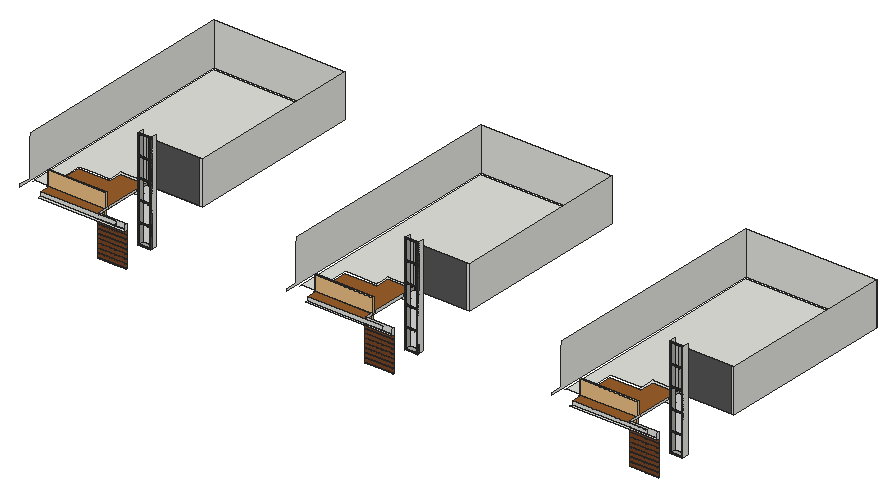
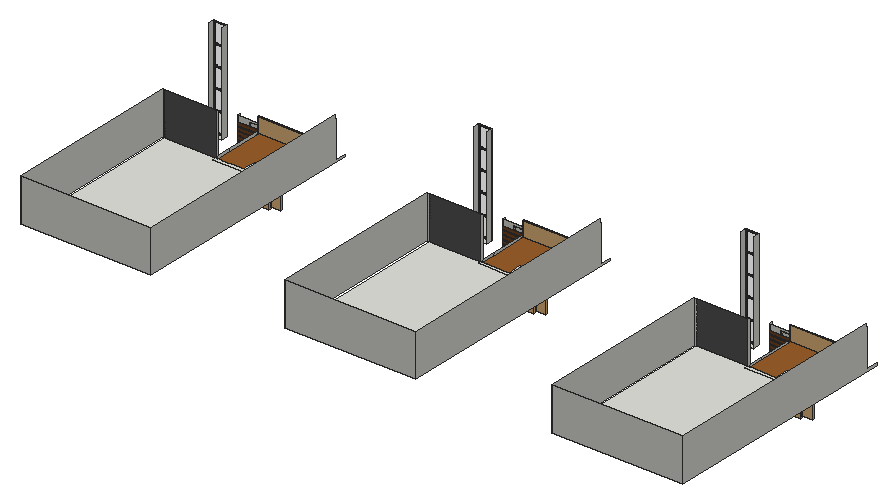
# SketchUp Ruby script. Lengths in inches.
U = 1.inch
M = Sketchup.active_model
def pt(a) = Geom::Point3d.new(a.map { |v| v * U })
def face(e, loops, mat)
  f = e.add_face(loops[0].map { |a| pt(a) })
  loops[1..].each { |l| e.add_face(l.map { |a| pt(a) }).erase! }
  f.material = f.back_material = mat if mat
  f
end
# faces: each face lists its corners as indices into pts; further lists are holes
def faces(e, pts, list, mat = nil) = list.each { |f| face(e, (f[0].is_a?(Array) ? f : [f]).map { |l| l.map { |i| pts[i] } }, mat) }
# xy, xz, yz: faces in a plane at the given z, y or x. An outline is a flat list of corners, or four numbers for a rectangle; further outlines are holes
def ring(l) = l.size == 4 ? [[l[0], l[1]], [l[2], l[1]], [l[2], l[3]], [l[0], l[3]]] : l.each_slice(2).to_a
def flat(e, list, mat, &to3) = list.each { |f| face(e, (f[0].is_a?(Array) ? f : [f]).map { |l| ring(l).map { |u, v| to3.(u, v) } }, mat) }
def xy(e, z, list, mat = nil) = flat(e, list, mat) { |x, y| [x, y, z] }
def xz(e, y, list, mat = nil) = flat(e, list, mat) { |x, z| [x, y, z] }
def yz(e, x, list, mat = nil) = flat(e, list, mat) { |y, z| [x, y, z] }
def lines(e, pts, list) = list.each { |a, b| e.add_line(pt(pts[a]), pt(pts[b])) }
# prism: a flat outline (further loops are holes) pulled along v
def prism(e, loops, v, mat = nil)
  f = face(e, loops, mat); d = Geom::Vector3d.new(v.map { |x| x * U })
  f.pushpull(f.normal.samedirection?(d) ? d.length : -d.length)
end
def box(e, o, s, mat = nil) = prism(e, [[o, [o[0] + s[0], o[1], o[2]], [o[0] + s[0], o[1] + s[1], o[2]], [o[0], o[1] + s[1], o[2]]]], [0, 0, s[2]], mat)
def at(x, y, z, deg = 0) = Geom::Transformation.translation(pt([x, y, z])) * Geom::Transformation.rotation(ORIGIN, Z_AXIS, deg.degrees)
def axes(o, x, y, z) = Geom::Transformation.new([*x, 0, *y, 0, *z, 0, *pt(o).to_a, 1])
def part(name) = M.definitions.add(name)
# library, detail: a bought-in or finely detailed component or shape, given as its bounding box
def library(name, o, s) = part(name).tap { |d| box(d.entities, o, s) }
def detail(e, o, s) = box(e.add_group.entities, o, s)
def put(e, d, t, mat = nil) = e.add_instance(d, t).tap { |i| i.material = mat if mat }
def group(e, t, mat = nil) = e.add_group.tap { |g| g.transformation = t; g.material = mat if mat }.entities
root = M.entities
M.materials.add("Aluminum_Polished").color = [83, 85, 85]
M.materials.add("Glass_Window_Neutral").color = [0, 0, 0]
M.materials["Glass_Window_Neutral"].alpha = 0.125
M.materials.add("[Color M04]").color = [142, 142, 142]
M.materials.add("[Color M06]").color = [86, 86, 86]
M.materials.add("[Wood Floor Dark]").color = [153, 94, 42]
M.materials.add("[Wood Veneer 01]").color = [120, 70, 37]
c1 = library("Group\#1",[0,0,0],[29.75,5.78,110.95])
c2 = part("Group\#54")
box(c2.entities,[0,0,0],[2,1,28])
c3 = part("Group\#56")
p = [[0.11,0.32,0.14],[0.11,0.69,0.14]]
lines(c3.entities,p,[[0,1]])
g1 = group(c3.entities,at(0.11,0,0))
prism(g1,[[[0,0.24,0],[0,0.32,0.14],[0,0.24,0.27],[0,0.08,0.27],[0,0,0.14],[0,0.08,0]]],[-0.11,0,0])
c4 = part("Ver Glass Railing")
g2 = group(c4.entities,at(0,0,0),"Aluminum_Polished")
box(g2,[0,0,0],[2,185,2])
g3 = group(c4.entities,at(0,0,2),"Aluminum_Polished")
p = [[1.41,1,0],[1.41,36.8,0],[1.41,184,0],[1.29,184,0],[1.29,1,0],[1.29,36.8,0],
  [1.41,184,28],[1.29,184,28],[1.41,148.2,28],[1.29,148.2,28],[1.41,1,28],[1.29,1,28],
  [1.29,111.4,28],[1.29,111.4,0],[1.41,111.4,0],[1.41,111.4,28],[1.29,110.4,0],[1.29,110.4,28],
  [1.41,110.4,28],[1.41,110.4,0],[1.29,74.6,28],[1.29,74.6,0],[1.41,74.6,0],[1.41,74.6,28],
  [1.29,73.6,0],[1.29,73.6,28],[1.41,73.6,28],[1.41,73.6,0],[1.29,148.2,0],[1.41,148.2,0],
  [1.29,147.2,0],[1.29,147.2,28],[1.41,147.2,28],[1.41,147.2,0],[1.29,37.8,28],[1.29,37.8,0],
  [1.41,37.8,0],[1.41,37.8,28],[1.29,36.8,28],[1.41,36.8,28]]
lines(g3,p,[[0,1],[2,3],[4,5],[6,7],[6,8],[7,9],[10,11],[2,6],[3,7],[0,4],[11,4],[10,0],
  [12,13],[14,15],[16,17],[18,19],[20,21],[22,23],[24,25],[26,27],[27,22],[24,21],[23,26],[20,25],
  [9,28],[29,8],[30,31],[32,33],[33,29],[30,28],[8,32],[9,31],[34,35],[36,37],[5,38],[39,1],
  [1,36],[5,35],[37,39],[14,33],[19,14],[22,19],[36,27],[13,30],[16,13],[21,16],[35,24],[15,18],
  [12,17],[29,2],[28,3],[18,23],[32,15],[17,20],[31,12],[26,37],[25,34],[34,38],[39,10],[38,11]])
g4 = group(g3,at(1.79,1,0))
box(g4,[-0.5,0,0],[0.125,183,28],"Glass_Window_Neutral")
g5 = group(g3,at(0,184,28))
box(g5,[0,-184,0],[2.5,185,1])
put(g3,c2,axes([2,185,28],[-1,0,0],[0,-1,0],[0,0,-1]))
put(g3,c2,axes([2,1,28],[-1,0,0],[0,-1,0],[0,0,-1]))
put(g3,c2,axes([2,111.4,28],[-1,0,0],[0,-1,0],[0,0,-1]))
put(g3,c2,axes([2,74.6,28],[-1,0,0],[0,-1,0],[0,0,-1]))
g6 = group(g3,at(2,148.2,28))
box(g6,[-2,-1,-28],[2,1,28])
put(g3,c2,axes([2,37.8,28],[-1,0,0],[0,-1,0],[0,0,-1]))
put(g3,c3,at(1.17,146.31,24.26))
put(g3,c3,axes([1.17,148.89,24.54],[1,0,0],[0,-1,0],[0,0,-1]))
put(g3,c3,axes([1.17,148.89,4.79],[1,0,0],[0,-1,0],[0,0,-1]))
put(g3,c3,at(1.17,146.31,4.51))
put(g3,c3,at(1.17,109.51,4.51))
put(g3,c3,axes([1.17,112.09,4.79],[1,0,0],[0,-1,0],[0,0,-1]))
put(g3,c3,axes([1.17,112.09,24.54],[1,0,0],[0,-1,0],[0,0,-1]))
put(g3,c3,at(1.17,109.51,24.26))
put(g3,c3,axes([1.17,75.29,24.54],[1,0,0],[0,-1,0],[0,0,-1]))
put(g3,c3,at(1.17,72.71,4.51))
put(g3,c3,axes([1.17,75.29,4.79],[1,0,0],[0,-1,0],[0,0,-1]))
put(g3,c3,at(1.17,72.71,24.26))
put(g3,c3,axes([1.17,38.49,24.54],[1,0,0],[0,-1,0],[0,0,-1]))
put(g3,c3,at(1.17,35.91,4.51))
put(g3,c3,axes([1.17,38.49,4.79],[1,0,0],[0,-1,0],[0,0,-1]))
put(g3,c3,at(1.17,35.91,24.26))
c5 = library("Glass Railing",[0,0,0],[139.5,4.76,42])
xy(root,154.375,[[1098.03,272.125,1148.06,273.0625],[1148.06,272.125,1181.97,273.0625],[1884.4,272.125,1934.43,273.0625],[1934.43,272.125,1968.34,273.0625],[2664.78,272.125,2714.81,273.0625],
  [2714.81,272.125,2748.72,273.0625]])
xy(root,155.86,[[1098.03,272.125,1181.97,273.0625],[1884.4,272.125,1968.34,273.0625],[2664.78,272.125,2748.72,273.0625]])
xy(root,167.1875,[[1098.03,272.125,1148.06,273.0625],[1148.06,272.125,1181.97,273.0625],[1884.4,272.125,1934.43,273.0625],[1934.43,272.125,1968.34,273.0625],[2664.78,272.125,2714.81,273.0625],
  [2714.81,272.125,2748.72,273.0625]])
xy(root,168.67,[[1098.03,272.125,1181.97,273.0625],[1884.4,272.125,1968.34,273.0625],[2664.78,272.125,2748.72,273.0625]])
xy(root,180,[[1098.03,272.125,1148.06,273.0625],[1148.06,272.125,1181.97,273.0625],[1884.4,272.125,1934.43,273.0625],[1934.43,272.125,1968.34,273.0625],[2664.78,272.125,2714.81,273.0625],
  [2714.81,272.125,2748.72,273.0625]])
xy(root,181.48,[[1098.03,272.125,1181.97,273.0625],[1884.4,272.125,1968.34,273.0625],[2664.78,272.125,2748.72,273.0625]])
xy(root,192.8125,[[1098.03,272.125,1148.06,273.0625],[1148.06,272.125,1181.97,273.0625],[1884.4,272.125,1934.43,273.0625],[1934.43,272.125,1968.34,273.0625],[2664.78,272.125,2714.81,273.0625],
  [2714.81,272.125,2748.72,273.0625]])
xy(root,194.3,[[1098.03,272.125,1181.97,273.0625],[1884.4,272.125,1968.34,273.0625],[2664.78,272.125,2748.72,273.0625]])
xy(root,205.625,[[1098.03,272.125,1148.06,273.0625],[1148.06,272.125,1181.97,273.0625],[1884.4,272.125,1934.43,273.0625],[1934.43,272.125,1968.34,273.0625],[2664.78,272.125,2714.81,273.0625],
  [2714.81,272.125,2748.72,273.0625]])
xy(root,207.11,[[1098.03,272.125,1181.97,273.0625],[1884.4,272.125,1968.34,273.0625],[2664.78,272.125,2748.72,273.0625]])
xy(root,217.36,[[1200.15,289.5,1239.03,308.24],[1986.53,289.5,2025.4,308.24],[2766.9,289.5,2805.78,308.24]])
xy(root,218.4375,[[1098.03,272.125,1148.06,273.0625],[1148.06,272.125,1181.97,273.0625],[1884.4,272.125,1934.43,273.0625],[1934.43,272.125,1968.34,273.0625],[2664.78,272.125,2714.81,273.0625],
  [2714.81,272.125,2748.72,273.0625]])
xy(root,219.92,[[1098.03,272.125,1181.97,273.0625],[1884.4,272.125,1968.34,273.0625],[2664.78,272.125,2748.72,273.0625]])
xy(root,231.25,[[1098.03,272.125,1148.06,273.0625],[1148.06,272.125,1181.97,273.0625],[1884.4,272.125,1934.43,273.0625],[1934.43,272.125,1968.34,273.0625],[2664.78,272.125,2714.81,273.0625],
  [2714.81,272.125,2748.72,273.0625]])
xy(root,231.75,[[1037.97,452.5625,1079.72,462.67],[1824.35,452.5625,1866.1,462.67],[2604.72,452.5625,2646.47,462.67]])
xy(root,232.73,[[1098.03,272.125,1181.97,273.0625],[1884.4,272.125,1968.34,273.0625],[2664.78,272.125,2748.72,273.0625]])
xy(root,244.0625,[[1098.03,272.125,1148.06,273.0625],[1148.06,272.125,1181.97,273.0625],[1884.4,272.125,1934.43,273.0625],[1934.43,272.125,1968.34,273.0625],[2664.78,272.125,2714.81,273.0625],
  [2714.81,272.125,2748.72,273.0625]])
xy(root,245.55,[[1098.03,272.125,1181.97,273.0625],[1884.4,272.125,1968.34,273.0625],[2664.78,272.125,2748.72,273.0625]])
xy(root,256.875,[[928.09,264.125,928.09,272.68,1098.03,272.98,1098.03,272.125,1181.97,272.125,1181.97,264.125],[1714.47,264.125,1714.47,272.68,1884.4,272.98,1884.4,272.125,1968.34,272.125,1968.34,264.125],[2494.84,264.125,2494.84,272.68,2664.78,272.98,2664.78,272.125,2748.72,272.125,2748.72,264.125],[1098.03,272.125,1098.03,272.98,1148.06,273.0625,1148.06,272.125],[1148.06,272.125,1181.97,273.0625],
  [1884.4,272.125,1884.4,272.98,1934.43,273.0625,1934.43,272.125],[1934.43,272.125,1968.34,273.0625],[2664.78,272.125,2664.78,272.98,2714.81,273.0625,2714.81,272.125],[2714.81,272.125,2748.72,273.0625],[1098.03,272.98,1148.06,273.0625,1098.03,273.0625],
  [1884.4,272.98,1934.43,273.0625,1884.4,273.0625],[2664.78,272.98,2714.81,273.0625,2664.78,273.0625]])
xy(root,267.625,[[881.96,308.24,922.07,308.24,922.07,421.04,971.61,421.04,1012.79,420.39,1012.79,462.67,1103.7,462.67,1103.7,452.5625,1253.34,452.5625,1253.34,968.69,881.96,968.69],[1668.33,308.24,1708.45,308.24,1708.45,421.04,1757.99,421.04,1799.16,420.39,1799.16,462.67,1890.08,462.67,1890.08,452.5625,2039.72,452.5625,2039.72,968.69,1668.33,968.69],[2448.71,308.24,2488.82,308.24,2488.82,421.04,2538.36,421.04,2579.54,420.39,2579.54,462.67,2670.45,462.67,2670.45,452.5625,2820.09,452.5625,2820.09,968.69,2448.71,968.69],[1012.79,411.0625,1019.84,411.0625,1019.84,452.5625,1103.7,452.5625,1103.7,462.67,1012.79,462.67],[1799.16,411.0625,1806.22,411.0625,1806.22,452.5625,1890.08,452.5625,1890.08,462.67,1799.16,462.67],
  [2579.54,411.0625,2586.59,411.0625,2586.59,452.5625,2670.45,452.5625,2670.45,462.67,2579.54,462.67]])
xy(root,267.625,[[928.09,272.68,928.09,411.0625,1019.84,411.0625,1019.84,452.5625,1098.03,452.5625,1098.03,273.0625,1148.06,273.0625],[1714.47,272.68,1714.47,411.0625,1806.22,411.0625,1806.22,452.5625,1884.4,452.5625,1884.4,273.0625,1934.43,273.0625],[2494.84,272.68,2494.84,411.0625,2586.59,411.0625,2586.59,452.5625,2664.78,452.5625,2664.78,273.0625,2714.81,273.0625]],"[Wood Floor Dark]")
xz(root,272.125,[[1098.03,155.86,1181.97,167.1875],[1884.4,155.86,1968.34,167.1875],[2664.78,155.86,2748.72,167.1875],[1098.03,168.67,1181.97,180],[1884.4,168.67,1968.34,180],
  [2664.78,168.67,2748.72,180],[1098.03,181.48,1181.97,192.8125],[1884.4,181.48,1968.34,192.8125],[2664.78,181.48,2748.72,192.8125],[1098.03,194.3,1181.97,205.625],
  [1884.4,194.3,1968.34,205.625],[2664.78,194.3,2748.72,205.625],[1098.03,207.11,1181.97,218.4375],[1884.4,207.11,1968.34,218.4375],[2664.78,207.11,2748.72,218.4375],
  [1098.03,219.92,1181.97,231.25],[1884.4,219.92,1968.34,231.25],[2664.78,219.92,2748.72,231.25],[1098.03,232.73,1181.97,244.0625],[1884.4,232.73,1968.34,244.0625],
  [2664.78,232.73,2748.72,244.0625],[1098.03,245.55,1181.97,256.875],[1884.4,245.55,1968.34,256.875],[2664.78,245.55,2748.72,256.875]],"[Wood Veneer 01]")
xz(root,273.0625,[[1098.03,256.875,1148.06,267.625],[1148.06,256.875,1181.97,256.875,1181.97,273.625,1098.03,273.625,1098.03,267.625,1148.06,267.625],[1884.4,256.875,1934.43,267.625],[1934.43,256.875,1968.34,256.875,1968.34,273.625,1884.4,273.625,1884.4,267.625,1934.43,267.625],[2664.78,256.875,2714.81,267.625],
  [2714.81,256.875,2748.72,256.875,2748.72,273.625,2664.78,273.625,2664.78,267.625,2714.81,267.625]])
xz(root,273.0625,[[1098.03,154.375,1181.97,155.86],[1884.4,154.375,1968.34,155.86],[2664.78,154.375,2748.72,155.86],[1098.03,167.1875,1181.97,168.67],[1884.4,167.1875,1968.34,168.67],
  [2664.78,167.1875,2748.72,168.67],[1098.03,180,1181.97,181.48],[1884.4,180,1968.34,181.48],[2664.78,180,2748.72,181.48],[1098.03,192.8125,1181.97,194.3],
  [1884.4,192.8125,1968.34,194.3],[2664.78,192.8125,2748.72,194.3],[1098.03,205.625,1181.97,207.11],[1884.4,205.625,1968.34,207.11],[2664.78,205.625,2748.72,207.11],
  [1098.03,218.4375,1181.97,219.92],[1884.4,218.4375,1968.34,219.92],[2664.78,218.4375,2748.72,219.92],[1098.03,231.25,1181.97,232.73],[1884.4,231.25,1968.34,232.73],
  [2664.78,231.25,2748.72,232.73],[1098.03,244.0625,1181.97,245.55],[1884.4,244.0625,1968.34,245.55],[2664.78,244.0625,2748.72,245.55]],"[Wood Veneer 01]")
xz(root,452.5625,[[1098.03,267.625,1103.7,393.625],[1253.34,267.625,1260.59,393.625],[1884.4,267.625,1890.08,393.625],[2039.72,267.625,2046.96,393.625],[2664.78,267.625,2670.45,393.625],
  [2820.09,267.625,2827.34,393.625]])
xz(root,452.5625,[[1103.7,267.625,1253.34,393.625],[1890.08,267.625,2039.72,393.625],[2670.45,267.625,2820.09,393.625]],"[Color M06]")
xz(root,975.9375,[[874.71,267.625,1260.59,393.625],[1661.09,267.625,2046.96,393.625],[2441.46,267.625,2827.34,393.625]])
yz(root,874.71,[[264.125,267.625,264.125,273.625,297.375,273.625,297.375,382.6875,301,382.6875,301,393.625,975.9375,393.625,975.9375,267.625]])
yz(root,1098.03,[[273.0625,267.625,308.24,273.625],[308.24,267.625,411.0625,273.625],[411.0625,267.625,452.5625,273.625]])
yz(root,1181.97,[[264.125,256.875,273.0625,273.625]])
yz(root,1200.15,[[289.5,217.36,308.24,512.23]])
yz(root,1239.03,[[289.5,217.36,308.24,512.23]])
yz(root,1260.59,[[452.5625,267.625,975.9375,393.625]])
yz(root,1661.09,[[264.125,267.625,264.125,273.625,297.375,273.625,297.375,382.6875,301,382.6875,301,393.625,975.9375,393.625,975.9375,267.625]])
yz(root,1884.4,[[273.0625,267.625,308.24,273.625],[308.24,267.625,411.0625,273.625],[411.0625,267.625,452.5625,273.625]])
yz(root,1968.34,[[264.125,256.875,273.0625,273.625]])
yz(root,1986.53,[[289.5,217.36,308.24,512.23]])
yz(root,2025.4,[[289.5,217.36,308.24,512.23]])
yz(root,2046.96,[[452.5625,267.625,975.9375,393.625]])
yz(root,2441.46,[[264.125,267.625,264.125,273.625,297.375,273.625,297.375,382.6875,301,382.6875,301,393.625,975.9375,393.625,975.9375,267.625]])
yz(root,2664.78,[[273.0625,267.625,308.24,273.625],[308.24,267.625,411.0625,273.625],[411.0625,267.625,452.5625,273.625]])
yz(root,2748.72,[[264.125,256.875,273.0625,273.625]])
yz(root,2766.9,[[289.5,217.36,308.24,512.23]])
yz(root,2805.78,[[289.5,217.36,308.24,512.23]])
yz(root,2827.34,[[452.5625,267.625,975.9375,393.625]])
p = [[928.09,272.68,267.625],[1148.06,273.0625,267.625],[1148.06,273.0625,256.875],[1098.03,272.98,256.875],[928.09,272.68,256.875],[1714.47,272.68,267.625],
  [1934.43,273.0625,267.625],[1934.43,273.0625,256.875],[1884.4,272.98,256.875],[1714.47,272.68,256.875],[2494.84,272.68,267.625],[2714.81,273.0625,267.625],
  [2714.81,273.0625,256.875],[2664.78,272.98,256.875],[2494.84,272.68,256.875],[1708.45,308.24,267.625],[1708.45,301,267.625],[1668.33,308.24,267.625],
  [1668.33,301,267.625],[922.07,308.24,267.625],[922.07,301,267.625],[881.96,308.24,267.625],[881.96,301,267.625],[2448.71,308.24,267.625],
  [2448.71,301,267.625],[2488.82,308.24,267.625],[2488.82,301,267.625]]
faces(root,p,[[0,1,2,3,4],[5,6,7,8,9],[10,11,12,13,14]])
lines(root,p,[[15,16],[17,18],[19,20],[21,22],[23,24],[25,26]])
put(root,c1,axes([1758.29,415.83,161.77],[1,0,0],[0,1,0],[0,0,0.62]),"[Color M04]")
put(root,c1,axes([971.91,415.83,161.77],[1,0,0],[0,1,0],[0,0,0.62]),"[Color M04]")
put(root,c1,axes([2538.66,415.83,161.77],[1,0,0],[0,1,0],[0,0,0.62]),"[Color M04]")
put(root,c1,axes([1723.6,415.83,171.76],[1,0,0],[0,1,0],[0,0,0.53]),"[Color M04]")
put(root,c1,axes([937.22,415.83,171.76],[1,0,0],[0,1,0],[0,0,0.53]),"[Color M04]")
put(root,c1,axes([2503.97,415.83,171.76],[1,0,0],[0,1,0],[0,0,0.53]),"[Color M04]")
put(root,c4,axes([2025.4,292,217.36],[0,-1,0],[0,0,1.59392],[-1.25403,0,0]))
put(root,c4,axes([1239.03,292,217.36],[0,-1,0],[0,0,1.59392],[-1.25403,0,0]))
put(root,c4,axes([2805.78,292,217.36],[0,-1,0],[0,0,1.59392],[-1.25403,0,0]))
put(root,c5,axes([1713.9,300.5625,271.02],[1.22225,0,0],[0,1,0],[0,0,1]))
put(root,c5,axes([927.52,300.5625,271.02],[1.22225,0,0],[0,1,0],[0,0,1]))
put(root,c5,axes([2494.27,300.5625,271.02],[1.22225,0,0],[0,1,0],[0,0,1]))
